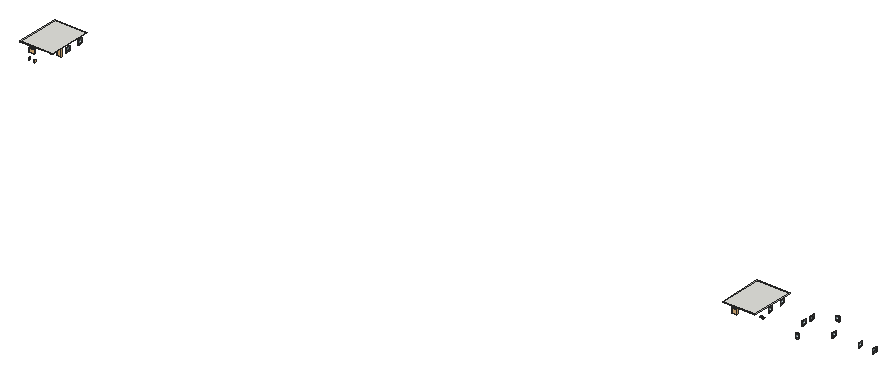
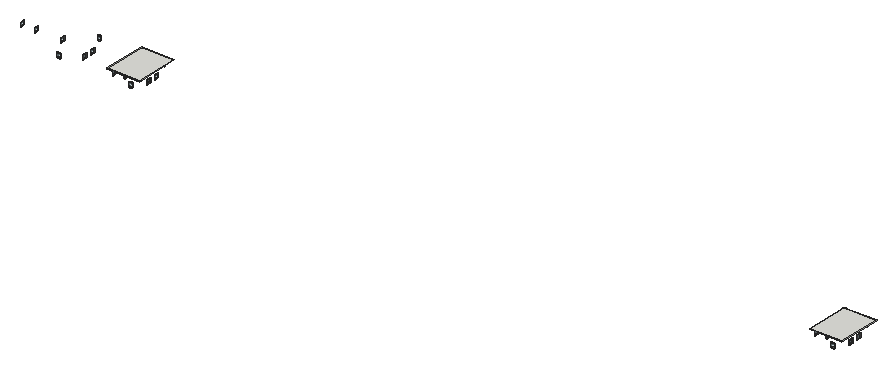
# SketchUp Ruby script. Lengths in inches.
U = 1.inch
M = Sketchup.active_model
def pt(a) = Geom::Point3d.new(a.map { |v| v * U })
def face(e, loops, mat)
  f = e.add_face(loops[0].map { |a| pt(a) })
  loops[1..].each { |l| e.add_face(l.map { |a| pt(a) }).erase! }
  f.material = f.back_material = mat if mat
  f
end
# faces: each face lists its corners as indices into pts; further lists are holes
def faces(e, pts, list, mat = nil) = list.each { |f| face(e, (f[0].is_a?(Array) ? f : [f]).map { |l| l.map { |i| pts[i] } }, mat) }
# xy, xz, yz: faces in a plane at the given z, y or x. An outline is a flat list of corners, or four numbers for a rectangle; further outlines are holes
def ring(l) = l.size == 4 ? [[l[0], l[1]], [l[2], l[1]], [l[2], l[3]], [l[0], l[3]]] : l.each_slice(2).to_a
def flat(e, list, mat, &to3) = list.each { |f| face(e, (f[0].is_a?(Array) ? f : [f]).map { |l| ring(l).map { |u, v| to3.(u, v) } }, mat) }
def xy(e, z, list, mat = nil) = flat(e, list, mat) { |x, y| [x, y, z] }
def xz(e, y, list, mat = nil) = flat(e, list, mat) { |x, z| [x, y, z] }
def yz(e, x, list, mat = nil) = flat(e, list, mat) { |y, z| [x, y, z] }
def lines(e, pts, list) = list.each { |a, b| e.add_line(pt(pts[a]), pt(pts[b])) }
# prism: a flat outline (further loops are holes) pulled along v
def prism(e, loops, v, mat = nil)
  f = face(e, loops, mat); d = Geom::Vector3d.new(v.map { |x| x * U })
  f.pushpull(f.normal.samedirection?(d) ? d.length : -d.length)
end
def box(e, o, s, mat = nil) = prism(e, [[o, [o[0] + s[0], o[1], o[2]], [o[0] + s[0], o[1] + s[1], o[2]], [o[0], o[1] + s[1], o[2]]]], [0, 0, s[2]], mat)
def at(x, y, z, deg = 0) = Geom::Transformation.translation(pt([x, y, z])) * Geom::Transformation.rotation(ORIGIN, Z_AXIS, deg.degrees)
def axes(o, x, y, z) = Geom::Transformation.new([*x, 0, *y, 0, *z, 0, *pt(o).to_a, 1])
def part(name) = M.definitions.add(name)
# library, detail: a bought-in or finely detailed component or shape, given as its bounding box
def library(name, o, s) = part(name).tap { |d| box(d.entities, o, s) }
def detail(e, o, s) = box(e.add_group.entities, o, s)
def put(e, d, t, mat = nil) = e.add_instance(d, t).tap { |i| i.material = mat if mat }
def group(e, t, mat = nil) = e.add_group.tap { |g| g.transformation = t; g.material = mat if mat }.entities
root = M.entities
M.materials.add("[Color M06]").color = [86, 86, 86]
M.materials.add("[Translucent Glass Safety]").color = [204, 235, 244]
M.materials["[Translucent Glass Safety]"].alpha = 0.5
M.materials.add("[Translucent_Glass_Gray]").color = [128, 128, 128]
M.materials["[Translucent_Glass_Gray]"].alpha = 0.5
c1 = library("A$C6E5D1AD4",[-33.75,-10.28,0],[67.5,20.56,0.01])
c2 = library("Indoor Plant 004",[-26.75,-21.09,0],[44.44,41.03,87.36])
c3 = library("Spot Light",[-5.1,-5.1,-11.05],[10.2,10.2,11.05])
c4 = library("Lamp Wall Outdoor 94-02",[-1.89,-4.65,-3.17],[3.78,4.65,6.35])
c5 = library("Door 243 065",[-19.36,-2.49,0],[38.72,4.98,81.96])
c6 = part("Group\#3")
xy(c6.entities,0,[[0,0,0.83,48],[0.83,0,2.5625,48]])
xy(c6.entities,3,[[0,3,0.67,45],[1.8,3,2.5625,45]])
xy(c6.entities,4.625,[[0.67,4.625,1.8,43.375]])
xy(c6.entities,43.375,[[0.67,4.625,1.8,43.375]])
xy(c6.entities,45,[[0,3,0.67,45],[1.8,3,2.5625,45]])
xy(c6.entities,48,[[0,0,0.83,48],[0.83,0,2.5625,48]])
xz(c6.entities,0,[[0,0,0.83,48],[0.83,0,2.5625,48]])
xz(c6.entities,3,[[0,3,0.67,45],[1.8,3,2.5625,45]])
xz(c6.entities,4.625,[[0.67,4.625,1.8,43.375]])
xz(c6.entities,43.375,[[0.67,4.625,1.8,43.375]])
xz(c6.entities,45,[[0,3,0.67,45],[1.8,3,2.5625,45]])
xz(c6.entities,48,[[0,0,0.83,48],[0.83,0,2.5625,48]])
yz(c6.entities,0,[[[0,0,48,48],[3,3,45,45]]])
yz(c6.entities,0.67,[[[3,3,45,45],[4.625,4.625,43.375,43.375]]])
yz(c6.entities,1.8,[[[3,3,45,45],[4.625,4.625,43.375,43.375]]])
yz(c6.entities,2.5625,[[[0,0,48,48],[3,3,45,45]]])
p = [[1.33,43.375,43.05],[1.33,43.375,4.66],[1.23,4.625,4.66],[1.23,4.625,43.05]]
faces(c6.entities,p,[[0,1,2,3]],"[Translucent Glass Safety]")
c7 = library("Window 109 011",[-27.22,-3.26,-0.09],[54.45,6.58,70.7])
c8 = part("Group\#7")
p = [[0,43.31,5.11],[2.95,43.31,0],[2.95,0,0],[0,0,5.11]]
faces(c8.entities,p,[[0,1,2,3]],"[Translucent_Glass_Gray]")
c9 = part("Vwntilation window")
put(c9.entities,c8,at(43.48,1.97,32.29))
put(c9.entities,c8,at(43.48,1.97,26.38))
put(c9.entities,c8,at(43.48,1.97,20.48))
put(c9.entities,c8,at(43.48,1.97,14.57))
put(c9.entities,c8,at(43.48,1.97,8.67))
put(c9.entities,c8,at(43.48,1.97,2.76))
g1 = group(c9.entities,at(43.48,0,0))
prism(g1,[[[1.97,47.24,39.37],[1.97,0,39.37],[1.97,0,0],[1.97,47.24,0]],[[1.97,45.28,1.97],[1.97,1.97,1.97],[1.97,1.97,37.4],[1.97,45.28,37.4]]],[-1.97,0,0])
c10 = part("Group\#8")
box(c10.entities,[0,-13.45,0],[366,489,4])
p = [[8188.44,830.24,100.75],[8188.44,878.24,100.75],[8188.44,878.24,52.75],[8188.44,830.24,52.75],[420.73,666.96,52.75],[420.73,618.96,52.75],
  [420.73,618.96,100.75],[420.73,666.96,100.75]]
lines(root,p,[[0,1],[1,2],[2,3],[3,0],[4,5],[6,7],[7,4],[5,6]])
put(root,c1,axes([8501.94,669.22,17.33],[0.71111,0,0],[0,0.71111,0],[0,0,0.71111]))
put(root,c2,axes([619.77,242.54,17.82],[0.28,0,0],[0,0.28,0],[0,0,0.28]))
put(root,c3,axes([559.3125,245.99,29.25],[0.66,0,0],[0,0.66,0],[0,0,0.66]))
put(root,c4,axes([559.3125,248.125,32.84],[1.4652,0,0],[0,0.66,0],[0,0,1.1286]))
put(root,c5,axes([734.18,452.17,30.68],[1.24138,0,0],[0,1.90527,0],[0,0,1.02567]))
put(root,c3,axes([559.59,246.34,36.41],[0.66,0,0],[0,-0.66,0],[0,0,-0.66]))
put(root,c6,at(498.73,777.1875,40.75,-90),"[Color M06]")
put(root,c6,at(8266.44,988.47,40.75,-90),"[Color M06]")
put(root,c7,axes([536.73,312.73,52.72],[1.10193,0,0],[0,1.87258,0],[0,0,0.6802]))
put(root,c7,axes([8304.45,524.01,52.72],[1.10193,0,0],[0,1.87258,0],[0,0,0.6802]))
put(root,c6,axes([9037.84,516.21,52.75],[0,1,0],[-0.75,0,0],[0,0,1]),"[Color M06]")
put(root,c6,at(424.4,618.96,52.75),"[Color M06]")
put(root,c6,at(8192.11,830.24,52.75),"[Color M06]")
put(root,c6,at(9079.87,983.97,52.75,-90),"[Color M06]")
put(root,c6,at(764.67,507.625,52.75),"[Color M06]")
put(root,c6,at(9254.5,718.9,52.75),"[Color M06]")
put(root,c6,at(8532.38,718.9,52.75),"[Color M06]")
put(root,c6,at(8915.06,830.24,52.75),"[Color M06]")
put(root,c6,at(764.67,678.7,52.75),"[Color M06]")
put(root,c6,at(8532.38,889.98,52.75),"[Color M06]")
put(root,c6,at(9711.44,718.9,52.75),"[Color M06]")
put(root,c6,at(425.23,507.625,52.75),"[Color M06]")
put(root,c6,at(8192.94,718.9,52.75),"[Color M06]")
put(root,c6,at(9549.44,718.9,52.75),"[Color M06]")
put(root,c6,at(8915.89,718.9,52.75),"[Color M06]")
put(root,c9,axes([606.0625,743.43,106.75],[0,0.67181,0],[-0.50965,0,0],[0,0,0.4572]))
put(root,c9,axes([8373.78,954.71,106.75],[0,0.67181,0],[-0.50965,0,0],[0,0,0.4572]))
put(root,c10,at(420.73,303.57,136.75))
put(root,c10,at(8188.44,514.85,136.75))
